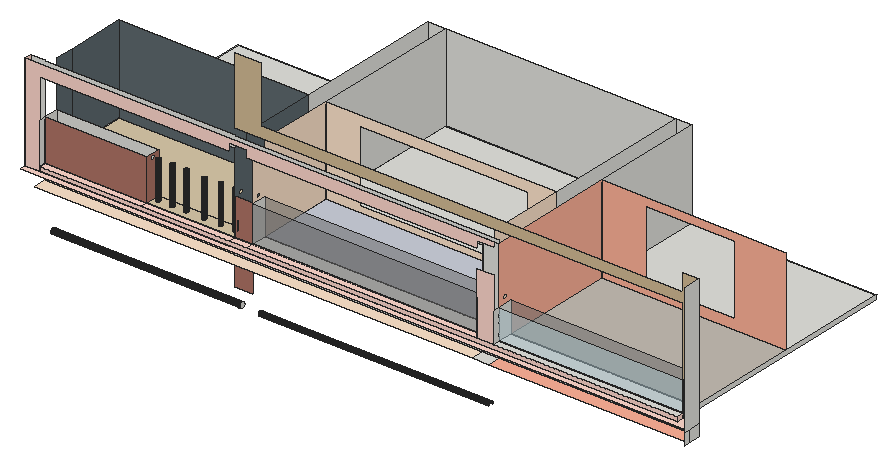
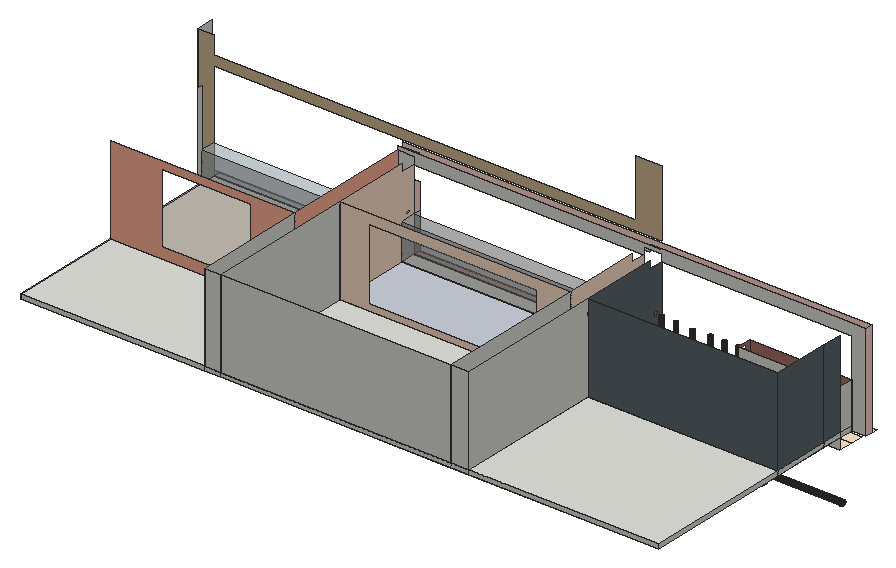
# SketchUp Ruby script. Lengths in inches.
U = 1.inch
M = Sketchup.active_model
def pt(a) = Geom::Point3d.new(a.map { |v| v * U })
def face(e, loops, mat)
  f = e.add_face(loops[0].map { |a| pt(a) })
  loops[1..].each { |l| e.add_face(l.map { |a| pt(a) }).erase! }
  f.material = f.back_material = mat if mat
  f
end
# faces: each face lists its corners as indices into pts; further lists are holes
def faces(e, pts, list, mat = nil) = list.each { |f| face(e, (f[0].is_a?(Array) ? f : [f]).map { |l| l.map { |i| pts[i] } }, mat) }
# xy, xz, yz: faces in a plane at the given z, y or x. An outline is a flat list of corners, or four numbers for a rectangle; further outlines are holes
def ring(l) = l.size == 4 ? [[l[0], l[1]], [l[2], l[1]], [l[2], l[3]], [l[0], l[3]]] : l.each_slice(2).to_a
def flat(e, list, mat, &to3) = list.each { |f| face(e, (f[0].is_a?(Array) ? f : [f]).map { |l| ring(l).map { |u, v| to3.(u, v) } }, mat) }
def xy(e, z, list, mat = nil) = flat(e, list, mat) { |x, y| [x, y, z] }
def xz(e, y, list, mat = nil) = flat(e, list, mat) { |x, z| [x, y, z] }
def yz(e, x, list, mat = nil) = flat(e, list, mat) { |y, z| [x, y, z] }
def lines(e, pts, list) = list.each { |a, b| e.add_line(pt(pts[a]), pt(pts[b])) }
# prism: a flat outline (further loops are holes) pulled along v
def prism(e, loops, v, mat = nil)
  f = face(e, loops, mat); d = Geom::Vector3d.new(v.map { |x| x * U })
  f.pushpull(f.normal.samedirection?(d) ? d.length : -d.length)
end
def box(e, o, s, mat = nil) = prism(e, [[o, [o[0] + s[0], o[1], o[2]], [o[0] + s[0], o[1] + s[1], o[2]], [o[0], o[1] + s[1], o[2]]]], [0, 0, s[2]], mat)
def at(x, y, z, deg = 0) = Geom::Transformation.translation(pt([x, y, z])) * Geom::Transformation.rotation(ORIGIN, Z_AXIS, deg.degrees)
def axes(o, x, y, z) = Geom::Transformation.new([*x, 0, *y, 0, *z, 0, *pt(o).to_a, 1])
def part(name) = M.definitions.add(name)
# library, detail: a bought-in or finely detailed component or shape, given as its bounding box
def library(name, o, s) = part(name).tap { |d| box(d.entities, o, s) }
def detail(e, o, s) = box(e.add_group.entities, o, s)
def put(e, d, t, mat = nil) = e.add_instance(d, t).tap { |i| i.material = mat if mat }
def group(e, t, mat = nil) = e.add_group.tap { |g| g.transformation = t; g.material = mat if mat }.entities
root = M.entities
M.materials.add("[Color B01]").color = [255, 216, 204]
M.materials.add("[Color B02]").color = [255, 178, 153]
M.materials.add("[Color C01]").color = [255, 229, 204]
M.materials.add("[Field Rectangle Tile]").color = [196, 189, 179]
M.materials.add("[Field Square Tile]").color = [217, 201, 169]
M.materials.add("[Formica Beige]").color = [211, 187, 149]
M.materials.add("[Formica Graystone]").color = [149, 146, 135]
M.materials.add("[Formica Laminate Dark]").color = [50, 53, 60]
M.materials.add("[Formica Speckled Grey]").color = [94, 105, 111]
M.materials.add("[Marble Carrara Floor Tile]").color = [204, 208, 219]
M.materials.add("[Stone Flagstone Ashlar]").color = [175, 116, 102]
M.materials.add("[Stone Flagstone Ashlar]1").color = [175, 116, 102]
M.materials.add("[Terrazzo Tile Light]").color = [219, 217, 210]
M.materials.add("[Translucent Glass Gray]").color = [128, 128, 128]
M.materials["[Translucent Glass Gray]"].alpha = 0.5
M.materials.add("[Translucent Glass Safety]").color = [204, 235, 244]
M.materials["[Translucent Glass Safety]"].alpha = 0.5
M.materials.add("[Wood Veneer 01]").color = [76, 44, 23]
xy(root,2054.4,[[2080.39,1246.93,2186.14,1258.93],[2207.95,1246.93,2312.17,1258.93]])
xy(root,2071.89,[[2062.91,1246.93,2329.66,1258.93]],"[Formica Laminate Dark]")
xy(root,2074.78,[[727.84,1144.55,801.89,1156.55],[817.41,1144.55,895.77,1156.55]])
xy(root,2077.28,[[1321.97,1144.55,1448.68,1156.55],[1465.17,1144.55,1591.81,1156.55],[1608.29,1144.55,1721.62,1156.55],[1738.1,1144.55,1854.25,1156.55]],"[Wood Veneer 01]")
xy(root,2083.5625,[[1905.54,863.74,1950.59,899.87]])
xy(root,2083.5625,[[1950.59,863.74,2507.95,899.87]],"[Color B02]")
xy(root,2083.5625,[[686.75,863.74,1905.54,899.87],[686.75,899.87,1950.59,941.93]],"[Color C01]")
xy(root,2089.12,[[713.49,1144.55,910.11,1156.55]])
xy(root,2092.65,[[1306.61,1144.55,1869.61,1156.55]])
xy(root,2114.125,[[646.49,880.68,686.75,899.87],[686.75,880.68,1214.63,899.87],[1214.63,880.68,1263.92,899.87],[1263.92,880.68,1905.54,899.87],[1905.54,880.68,1950.59,899.87],
  [1950.59,880.68,2463.34,899.87],[686.75,899.87,1214.63,941.93],[1214.63,899.87,1263.92,941.93],[1263.92,899.87,1905.54,941.93],[1905.54,899.87,1950.59,941.93],
  [1214.63,941.93,1263.92,1358.15],[1905.54,941.93,1950.59,1358.15],[686.75,1156.55,1214.63,1571.68],[1263.92,1156.55,1905.54,1358.15],[1950.59,1258.93,2463.34,1358.15],
  [1214.63,1358.15,1263.92,1571.68],[1263.92,1358.15,1905.54,1571.68],[1905.54,1358.15,1950.59,1571.68],[1950.59,1358.15,2463.34,1571.68]])
xy(root,2114.125,[[646.49,863.74,2507.95,863.74,2507.95,899.87,2463.34,899.87,2463.34,880.68,646.49,880.68]],"[Color B01]")
xy(root,2114.125,[[1950.59,899.87,2463.34,1258.93]],"[Color B02]")
xy(root,2114.125,[[1263.92,941.93,1905.54,1156.55]],"[Color C01]")
xy(root,2114.125,[[686.75,941.93,1214.63,1156.55]],"[Terrazzo Tile Light]")
xy(root,2126.125,[[1905.54,880.68,1950.59,899.87],[1950.59,880.68,2463.34,899.87],[686.75,899.87,969.66,941.93],[1214.63,899.87,1263.92,1571.68],[1263.92,899.87,1905.54,941.93],
  [1905.54,899.87,1950.59,1571.68],[1950.59,899.87,2463.34,941.93],[982.87,919.11,981.55,919.29,980.31,919.8,979.25,920.61,978.43,921.68,977.92,922.91,977.75,924.24,977.92,925.57,978.43,926.8,979.25,927.86,980.31,928.68,981.55,929.1875,982.87,929.36,984.2,929.1875,985.43,928.68,986.5,927.86,987.31,926.8,987.82,925.57,988,924.24,987.82,922.91,987.31,921.68,986.5,920.61,985.43,919.8,984.2,919.29],[1021.75,919.11,1020.42,919.29,1019.18,919.8,1018.12,920.61,1017.31,921.68,1016.8,922.91,1016.62,924.24,1016.8,925.57,1017.31,926.8,1018.12,927.86,1019.18,928.68,1020.42,929.1875,1021.75,929.36,1023.07,929.1875,1024.31,928.68,1025.37,927.86,1026.18,926.8,1026.7,925.57,1026.87,924.24,1026.7,922.91,1026.18,921.68,1025.37,920.61,1024.31,919.8,1023.07,919.29],[1060.43,919.11,1059.11,919.29,1057.87,919.8,1056.81,920.61,1056,921.68,1055.48,922.91,1055.31,924.24,1055.48,925.57,1056,926.8,1056.81,927.86,1057.87,928.68,1059.11,929.1875,1060.43,929.36,1061.76,929.1875,1063,928.68,1064.06,927.86,1064.87,926.8,1065.38,925.57,1065.56,924.24,1065.38,922.91,1064.87,921.68,1064.06,920.61,1063,919.8,1061.76,919.29],
  [1110.56,919.11,1109.23,919.29,1108,919.8,1106.94,920.61,1106.12,921.68,1105.61,922.91,1105.43,924.24,1105.61,925.57,1106.12,926.8,1106.94,927.86,1108,928.68,1109.23,929.1875,1110.56,929.36,1111.89,929.1875,1113.12,928.68,1114.18,927.86,1115,926.8,1115.51,925.57,1115.68,924.24,1115.51,922.91,1115,921.68,1114.18,920.61,1113.12,919.8,1111.89,919.29],[1156.68,919.11,1155.36,919.29,1154.12,919.8,1153.06,920.61,1152.25,921.68,1151.73,922.91,1151.56,924.24,1151.73,925.57,1152.25,926.8,1153.06,927.86,1154.12,928.68,1155.36,929.1875,1156.68,929.36,1158.01,929.1875,1159.25,928.68,1160.31,927.86,1161.12,926.8,1161.63,925.57,1161.81,924.24,1161.63,922.91,1161.12,921.68,1160.31,920.61,1159.25,919.8,1158.01,919.29],[1197.43,919.11,1196.11,919.29,1194.87,919.8,1193.81,920.61,1193,921.68,1192.48,922.91,1192.31,924.24,1192.48,925.57,1193,926.8,1193.81,927.86,1194.87,928.68,1196.11,929.1875,1197.43,929.36,1198.76,929.1875,1200,928.68,1201.06,927.86,1201.87,926.8,1202.38,925.57,1202.56,924.24,1202.38,922.91,1201.87,921.68,1201.06,920.61,1200,919.8,1198.76,919.29],[686.75,1156.55,1214.63,1571.68],[1263.92,1156.55,1905.54,1571.68],
  [1950.59,1258.05,2463.34,1571.68],[2463.34,1258.05,2464.28,1571.68]])
xy(root,2126.125,[[686.75,880.68,969.66,899.87],[969.66,880.68,1214.63,899.87],[1214.63,880.68,1263.92,899.87],[1263.92,880.68,1905.54,899.87]],"[Color B01]")
xy(root,2126.125,[[1950.59,941.93,2463.34,1258.05]],"[Field Rectangle Tile]")
xy(root,2126.125,[[[969.66,899.87,1214.63,941.93],[982.87,919.11,981.55,919.29,980.31,919.8,979.25,920.61,978.43,921.68,977.92,922.91,977.75,924.24,977.92,925.57,978.43,926.8,979.25,927.86,980.31,928.68,981.55,929.1875,982.87,929.36,984.2,929.1875,985.43,928.68,986.5,927.86,987.31,926.8,987.82,925.57,988,924.24,987.82,922.91,987.31,921.68,986.5,920.61,985.43,919.8,984.2,919.29],[1197.43,919.11,1196.11,919.29,1194.87,919.8,1193.81,920.61,1193,921.68,1192.48,922.91,1192.31,924.24,1192.48,925.57,1193,926.8,1193.81,927.86,1194.87,928.68,1196.11,929.1875,1197.43,929.36,1198.76,929.1875,1200,928.68,1201.06,927.86,1201.87,926.8,1202.38,925.57,1202.56,924.24,1202.38,922.91,1201.87,921.68,1201.06,920.61,1200,919.8,1198.76,919.29],[1021.75,919.11,1020.42,919.29,1019.18,919.8,1018.12,920.61,1017.31,921.68,1016.8,922.91,1016.62,924.24,1016.8,925.57,1017.31,926.8,1018.12,927.86,1019.18,928.68,1020.42,929.1875,1021.75,929.36,1023.07,929.1875,1024.31,928.68,1025.37,927.86,1026.18,926.8,1026.7,925.57,1026.87,924.24,1026.7,922.91,1026.18,921.68,1025.37,920.61,1024.31,919.8,1023.07,919.29],[1156.68,919.11,1155.36,919.29,1154.12,919.8,1153.06,920.61,1152.25,921.68,1151.73,922.91,1151.56,924.24,1151.73,925.57,1152.25,926.8,1153.06,927.86,1154.12,928.68,1155.36,929.1875,1156.68,929.36,1158.01,929.1875,1159.25,928.68,1160.31,927.86,1161.12,926.8,1161.63,925.57,1161.81,924.24,1161.63,922.91,1161.12,921.68,1160.31,920.61,1159.25,919.8,1158.01,919.29],[1060.43,919.11,1059.11,919.29,1057.87,919.8,1056.81,920.61,1056,921.68,1055.48,922.91,1055.31,924.24,1055.48,925.57,1056,926.8,1056.81,927.86,1057.87,928.68,1059.11,929.1875,1060.43,929.36,1061.76,929.1875,1063,928.68,1064.06,927.86,1064.87,926.8,1065.38,925.57,1065.56,924.24,1065.38,922.91,1064.87,921.68,1064.06,920.61,1063,919.8,1061.76,919.29],[1110.56,919.11,1109.23,919.29,1108,919.8,1106.94,920.61,1106.12,921.68,1105.61,922.91,1105.43,924.24,1105.61,925.57,1106.12,926.8,1106.94,927.86,1108,928.68,1109.23,929.1875,1110.56,929.36,1111.89,929.1875,1113.12,928.68,1114.18,927.86,1115,926.8,1115.51,925.57,1115.68,924.24,1115.51,922.91,1115,921.68,1114.18,920.61,1113.12,919.8,1111.89,919.29]],[686.75,941.93,1214.63,1156.55]],"[Field Square Tile]")
xy(root,2126.125,[[1263.92,941.93,1905.54,1156.55]],"[Marble Carrara Floor Tile]")
xz(root,880.68,[[646.49,2114.125,686.75,2114.125,686.75,2350.0625,1214.63,2350.0625,1214.63,2369.6875,1263.92,2369.6875,1263.92,2350.0625,1905.54,2350.0625,1905.54,2369.6875,1950.59,2369.6875,1950.59,2383.06,646.49,2383.06],[686.75,2114.125,2463.34,2126.125],[1905.54,2126.125,1950.59,2298.64]],"[Color B01]")
xz(root,899.87,[[1214.63,2083.5625,1263.92,2114.125],[1263.92,2083.5625,1905.54,2114.125],[1905.54,2083.5625,1950.59,2114.125],[1950.59,2083.5625,2463.34,2114.125],[2463.34,2083.5625,2507.95,2114.125],
  [646.49,2114.125,646.49,2383.06,686.75,2383.06,686.75,2381.6875,1215.84,2381.6875,1215.84,2379.45,1950.59,2379.45,1950.59,2369.6875,1905.54,2369.6875,1905.54,2350.0625,1263.92,2350.0625,1263.92,2369.6875,1214.63,2369.6875,1214.63,2350.0625,686.75,2350.0625,686.75,2114.125],[686.75,2114.125,2463.34,2126.125],[1905.54,2126.125,1950.59,2369.6875]])
xz(root,899.87,[[2463.34,2114.125,2507.95,2114.125,2507.95,2476.875,2463.34,2476.875,2463.34,2428.82,1286.83,2428.82,1286.83,2588.07,1215.84,2588.07,1215.84,2400.95,2463.34,2400.95]],"[Formica Beige]")
xz(root,899.87,[[686.75,2126.125,969.66,2241]],"[Stone Flagstone Ashlar]")
xz(root,899.87,[[1214.63,2003.5,1263.92,2083.5625],[1214.63,2126.125,1263.92,2230.66]],"[Stone Flagstone Ashlar]1")
xz(root,899.87,[[1263.92,2126.125,1905.54,2226.5]],"[Translucent Glass Gray]")
xz(root,899.87,[[1950.59,2126.125,2463.34,2209.0625]],"[Translucent Glass Safety]")
xz(root,941.93,[[686.75,2083.5625,1950.59,2114.125],[686.75,2126.125,969.66,2241]])
xz(root,941.93,[[1263.92,2126.125,1905.54,2226.5],[1950.59,2126.125,2463.34,2209.0625]],"[Translucent Glass Gray]")
xz(root,1156.55,[[[1263.92,2126.125,1905.54,2369.6875],[1358.7,2142.09,1824.89,2342.28]]],"[Color C01]")
xz(root,1156.55,[[686.75,2126.125,1214.63,2369.6875]],"[Formica Speckled Grey]")
xz(root,1258.05,[[[1950.59,2126.125,2464.28,2369.6875],[2073.08,2155.2,2321.89,2349.01]]],"[Color B02]")
xz(root,1571.68,[[686.75,2114.125,1214.63,2126.125],[1214.63,2114.125,1263.92,2126.125],[1263.92,2114.125,1905.54,2126.125],[1905.54,2114.125,1950.59,2126.125],[1950.59,2114.125,2463.34,2126.125],
  [1214.63,2126.125,1263.92,2369.6875],[1263.92,2126.125,1905.54,2369.6875],[1905.54,2126.125,1950.59,2369.6875]])
yz(root,646.49,[[880.68,2114.125,899.87,2383.06]],"[Color B01]")
yz(root,686.75,[[880.68,2114.125,899.87,2126.125],[899.87,2114.125,941.93,2126.125],[941.93,2114.125,994.87,2126.125],[994.87,2114.125,1156.55,2126.125],[1156.55,2114.125,1571.68,2126.125],
  [880.68,2126.125,899.87,2241],[899.87,2126.125,941.93,2241]])
yz(root,686.75,[[941.93,2126.125,994.87,2369.6875],[994.87,2126.125,1156.55,2369.6875]],"[Formica Speckled Grey]")
yz(root,969.66,[[[899.87,2126.125,941.93,2241],[921.12,2224.46,919.47,2224.68,917.93,2225.3125,916.61,2226.33,915.6,2227.65,914.96,2229.19,914.74,2230.84,914.96,2232.49,915.6,2234.02,916.61,2235.34,917.93,2236.36,919.47,2236.99,921.12,2237.21,922.77,2236.99,924.3,2236.36,925.625,2235.34,926.64,2234.02,927.27,2232.49,927.49,2230.84,927.27,2229.19,926.64,2227.65,925.625,2226.33,924.3,2225.3125,922.77,2224.68]]],"[Stone Flagstone Ashlar]")
yz(root,1214.63,[[927.21,1938.33,928.92,1938.56,930.51,1939.22,931.88,1940.26,932.93,1941.63,933.59,1943.22,933.8125,1944.93,933.59,1946.64,932.93,1948.23,931.88,1949.6,930.51,1950.65,928.92,1951.31,927.21,1951.53,925.5,1951.31,923.91,1950.65,922.55,1949.6,921.5,1948.23,920.84,1946.64,920.61,1944.93,920.84,1943.22,921.5,1941.63,922.55,1940.26,923.91,1939.22,925.5,1938.56],[1156.55,2126.125,1571.68,2369.6875]])
yz(root,1214.63,[[[899.87,2126.125,899.87,2350.0625,941.93,2350.0625,941.93,2369.6875,1156.55,2369.6875,1156.55,2126.125],[921.12,2224.46,922.77,2224.68,924.3,2225.3125,925.625,2226.33,926.64,2227.65,927.27,2229.19,927.49,2230.84,927.27,2232.49,926.64,2234.02,925.625,2235.34,924.3,2236.36,922.77,2236.99,921.12,2237.21,919.47,2236.99,917.93,2236.36,916.61,2235.34,915.6,2234.02,914.96,2232.49,914.74,2230.84,914.96,2229.19,915.6,2227.65,916.61,2226.33,917.93,2225.3125,919.47,2224.68]]],"[Formica Speckled Grey]")
yz(root,1263.92,[[899.87,2126.125,941.93,2226.5],[1156.55,2126.125,1571.68,2369.6875]])
yz(root,1263.92,[[[941.93,2126.125,1156.55,2126.125,1156.55,2369.6875,941.93,2369.6875,941.93,2350.0625,899.87,2350.0625,899.87,2226.5,941.93,2226.5],[920.9,2234.39,919.46,2234.58,918.12,2235.14,916.97,2236.02,916.08,2237.18,915.53,2238.52,915.34,2239.96,915.53,2241.4,916.08,2242.74,916.97,2243.89,918.12,2244.77,919.46,2245.33,920.9,2245.52,922.34,2245.33,923.68,2244.77,924.83,2243.89,925.72,2242.74,926.27,2241.4,926.46,2239.96,926.27,2238.52,925.72,2237.18,924.83,2236.02,923.68,2235.14,922.34,2234.58]]],"[Color C01]")
yz(root,1905.54,[[880.68,2126.125,899.87,2226.5],[899.87,2126.125,941.93,2226.5],[1156.55,2126.125,1571.68,2369.6875]])
yz(root,1905.54,[[[941.93,2126.125,941.93,2226.5,899.87,2226.5,899.87,2350.0625,941.93,2350.0625,941.93,2369.6875,1156.55,2369.6875,1156.55,2126.125],[920.9,2234.39,922.34,2234.58,923.68,2235.14,924.83,2236.02,925.72,2237.18,926.27,2238.52,926.46,2239.96,926.27,2241.4,925.72,2242.74,924.83,2243.89,923.68,2244.77,922.34,2245.33,920.9,2245.52,919.46,2245.33,918.12,2244.77,916.97,2243.89,916.08,2242.74,915.53,2241.4,915.34,2239.96,915.53,2238.52,916.08,2237.18,916.97,2236.02,918.12,2235.14,919.46,2234.58]]],"[Color C01]")
yz(root,1950.59,[[899.87,2083.5625,941.93,2114.125],[880.68,2126.125,899.87,2209.0625],[899.87,2126.125,941.93,2209.0625],[1258.05,2126.125,1571.68,2369.6875]])
yz(root,1950.59,[[[941.93,2126.125,1258.05,2126.125,1258.05,2369.6875,899.87,2369.6875,899.87,2209.0625,941.93,2209.0625],[920.9,2220.96,919.11,2221.2,917.43,2221.89,916,2222.99,914.89,2224.43,914.2,2226.1,913.96,2227.9,914.2,2229.69,914.89,2231.37,916,2232.8,917.43,2233.91,919.11,2234.6,920.9,2234.84,922.7,2234.6,924.37,2233.91,925.81,2232.8,926.91,2231.37,927.6,2229.69,927.84,2227.9,927.6,2226.1,926.91,2224.43,925.81,2222.99,924.37,2221.89,922.7,2221.2]]],"[Color B02]")
yz(root,2463.34,[[899.87,2114.125,941.93,2126.125],[941.93,2114.125,954.56,2126.125],[954.56,2114.125,1571.68,2126.125],[899.87,2126.125,941.93,2209.0625],[941.93,2126.125,954.56,2369.6875]])
yz(root,2463.34,[[880.68,2114.125,899.87,2126.125]],"[Color B01]")
yz(root,2507.95,[[849.3125,2083.5625,863.74,2114.125],[863.74,2083.5625,899.87,2114.125],[849.3125,2114.125,899.87,2476.875]])
p = [[1214.63,927.21,1938.33],[1214.63,925.5,1938.56],[686.75,925.5,1938.56],[686.75,927.21,1938.33],[1214.63,928.92,1938.56],[686.75,928.92,1938.56],
  [1214.63,923.91,1939.22],[686.75,923.91,1939.22],[1214.63,930.51,1939.22],[686.75,930.51,1939.22],[1905.54,920.8125,1939.12],[1905.54,920.59,1940.84],
  [1263.92,920.59,1940.84],[1263.92,920.8125,1939.12],[1905.54,933.84,1940.84],[1905.54,933.61,1939.12],[1263.92,933.61,1939.12],[1263.92,933.84,1940.84],
  [1214.63,922.55,1940.26],[686.75,922.55,1940.26],[1214.63,931.88,1940.26],[686.75,931.88,1940.26],[1214.63,921.5,1941.63],[686.75,921.5,1941.63],
  [1214.63,932.93,1941.63],[686.75,932.93,1941.63],[1905.54,920.8125,1942.55],[1263.92,920.8125,1942.55],[1905.54,933.61,1942.55],[1263.92,933.61,1942.55],
  [1214.63,920.84,1943.22],[686.75,920.84,1943.22],[1214.63,933.59,1943.22],[686.75,933.59,1943.22],[1905.54,921.48,1944.15],[1263.92,921.48,1944.15],
  [1905.54,932.95,1944.15],[1263.92,932.95,1944.15],[1214.63,920.61,1944.93],[686.75,920.61,1944.93],[1214.63,933.8125,1944.93],[686.75,933.8125,1944.93],
  [1905.54,922.53,1945.52],[1263.92,922.53,1945.52],[1905.54,931.9,1945.52],[1263.92,931.9,1945.52],[1214.63,920.84,1946.64],[686.75,920.84,1946.64],
  [1214.63,933.59,1946.64],[686.75,933.59,1946.64],[1905.54,923.9,1946.57],[1263.92,923.9,1946.57],[1905.54,930.53,1946.57],[1263.92,930.53,1946.57],
  [1214.63,921.5,1948.23],[686.75,921.5,1948.23],[1905.54,925.5,1947.24],[1263.92,925.5,1947.24],[1905.54,928.93,1947.24],[1263.92,928.93,1947.24],
  [1214.63,932.93,1948.23],[686.75,932.93,1948.23],[1905.54,927.21,1947.46],[1263.92,927.21,1947.46],[1214.63,922.55,1949.6],[686.75,922.55,1949.6],
  [1214.63,931.88,1949.6],[686.75,931.88,1949.6],[1214.63,923.91,1950.65],[686.75,923.91,1950.65],[1214.63,930.51,1950.65],[686.75,930.51,1950.65],
  [1214.63,925.5,1951.31],[686.75,925.5,1951.31],[1214.63,928.92,1951.31],[686.75,928.92,1951.31],[1214.63,927.21,1951.53],[686.75,927.21,1951.53],
  [981.55,919.29,2126.125],[982.87,919.11,2126.125],[982.87,919.11,2230.84],[981.55,919.29,2230.84],[984.2,919.29,2126.125],[984.2,919.29,2230.84],
  [1020.42,919.29,2126.125],[1021.75,919.11,2126.125],[1021.75,919.11,2230.84],[1020.42,919.29,2230.84],[1023.07,919.29,2126.125],[1023.07,919.29,2230.84],
  [1059.11,919.29,2126.125],[1060.43,919.11,2126.125],[1060.43,919.11,2230.84],[1059.11,919.29,2230.84],[1061.76,919.29,2126.125],[1061.76,919.29,2230.84],
  [1109.23,919.29,2126.125],[1110.56,919.11,2126.125],[1110.56,919.11,2228],[1109.23,919.29,2228],[1111.89,919.29,2126.125],[1111.89,919.29,2228],
  [1155.36,919.29,2126.125],[1156.68,919.11,2126.125],[1156.68,919.11,2230.84],[1155.36,919.29,2230.84],[1158.01,919.29,2126.125],[1158.01,919.29,2230.84],
  [1196.11,919.29,2126.125],[1197.43,919.11,2126.125],[1197.43,919.11,2232],[1196.11,919.29,2232],[1198.76,919.29,2126.125],[1198.76,919.29,2232],
  [980.31,919.8,2126.125],[980.31,919.8,2230.84],[985.43,919.8,2126.125],[985.43,919.8,2230.84],[1019.18,919.8,2126.125],[1019.18,919.8,2230.84],
  [1024.31,919.8,2126.125],[1024.31,919.8,2230.84],[1057.87,919.8,2126.125],[1057.87,919.8,2230.84],[1063,919.8,2126.125],[1063,919.8,2230.84],
  [1108,919.8,2126.125],[1108,919.8,2228],[1113.12,919.8,2126.125],[1113.12,919.8,2228],[1154.12,919.8,2126.125],[1154.12,919.8,2230.84],
  [1159.25,919.8,2126.125],[1159.25,919.8,2230.84],[1194.87,919.8,2126.125],[1194.87,919.8,2232],[1200,919.8,2126.125],[1200,919.8,2232],
  [979.25,920.61,2126.125],[979.25,920.61,2230.84],[986.5,920.61,2126.125],[986.5,920.61,2230.84],[1018.12,920.61,2126.125],[1018.12,920.61,2230.84],
  [1025.37,920.61,2126.125],[1025.37,920.61,2230.84],[1056.81,920.61,2126.125],[1056.81,920.61,2230.84],[1064.06,920.61,2126.125],[1064.06,920.61,2230.84],
  [1106.94,920.61,2126.125],[1106.94,920.61,2228],[1114.18,920.61,2126.125],[1114.18,920.61,2228],[1153.06,920.61,2126.125],[1153.06,920.61,2230.84],
  [1160.31,920.61,2126.125],[1160.31,920.61,2230.84],[1193.81,920.61,2126.125],[1193.81,920.61,2232],[1201.06,920.61,2126.125],[1201.06,920.61,2232],
  [978.43,921.68,2126.125],[978.43,921.68,2230.84],[987.31,921.68,2126.125],[987.31,921.68,2230.84],[1017.31,921.68,2126.125],[1017.31,921.68,2230.84],
  [1026.18,921.68,2126.125],[1026.18,921.68,2230.84],[1056,921.68,2126.125],[1056,921.68,2230.84],[1064.87,921.68,2126.125],[1064.87,921.68,2230.84],
  [1106.12,921.68,2126.125],[1106.12,921.68,2228],[1115,921.68,2126.125],[1115,921.68,2228],[1152.25,921.68,2126.125],[1152.25,921.68,2230.84],
  [1161.12,921.68,2126.125],[1161.12,921.68,2230.84],[1193,921.68,2126.125],[1193,921.68,2232],[1201.87,921.68,2126.125],[1201.87,921.68,2232],
  [977.92,922.91,2126.125],[977.92,922.91,2230.84],[987.82,922.91,2126.125],[987.82,922.91,2230.84],[1016.8,922.91,2126.125],[1016.8,922.91,2230.84],
  [1026.7,922.91,2126.125],[1026.7,922.91,2230.84],[1055.48,922.91,2126.125],[1055.48,922.91,2230.84],[1065.38,922.91,2126.125],[1065.38,922.91,2230.84],
  [1105.61,922.91,2126.125],[1105.61,922.91,2228],[1115.51,922.91,2126.125],[1115.51,922.91,2228],[1151.73,922.91,2126.125],[1151.73,922.91,2230.84],
  [1161.63,922.91,2126.125],[1161.63,922.91,2230.84],[1192.48,922.91,2126.125],[1192.48,922.91,2232],[1202.38,922.91,2126.125],[1202.38,922.91,2232],
  [977.75,924.24,2126.125],[977.75,924.24,2230.84],[988,924.24,2126.125],[988,924.24,2230.84],[1016.62,924.24,2126.125],[1016.62,924.24,2230.84],
  [1026.87,924.24,2126.125],[1026.87,924.24,2230.84],[1055.31,924.24,2126.125],[1055.31,924.24,2230.84],[1065.56,924.24,2126.125],[1065.56,924.24,2230.84],
  [1105.43,924.24,2126.125],[1105.43,924.24,2228],[1115.68,924.24,2126.125],[1115.68,924.24,2228],[1151.56,924.24,2126.125],[1151.56,924.24,2230.84],
  [1161.81,924.24,2126.125],[1161.81,924.24,2230.84],[1192.31,924.24,2126.125],[1192.31,924.24,2232],[1202.56,924.24,2126.125],[1202.56,924.24,2232],
  [977.92,925.57,2126.125],[977.92,925.57,2230.84],[987.82,925.57,2126.125],[987.82,925.57,2230.84],[1016.8,925.57,2126.125],[1016.8,925.57,2230.84],
  [1026.7,925.57,2126.125],[1026.7,925.57,2230.84],[1055.48,925.57,2126.125],[1055.48,925.57,2230.84],[1065.38,925.57,2126.125],[1065.38,925.57,2230.84],
  [1105.61,925.57,2126.125],[1105.61,925.57,2228],[1115.51,925.57,2126.125],[1115.51,925.57,2228],[1151.73,925.57,2126.125],[1151.73,925.57,2230.84],
  [1161.63,925.57,2126.125],[1161.63,925.57,2230.84],[1192.48,925.57,2126.125],[1192.48,925.57,2232],[1202.38,925.57,2126.125],[1202.38,925.57,2232],
  [978.43,926.8,2126.125],[978.43,926.8,2230.84],[987.31,926.8,2126.125],[987.31,926.8,2230.84],[1017.31,926.8,2126.125],[1017.31,926.8,2230.84],
  [1026.18,926.8,2126.125],[1026.18,926.8,2230.84],[1056,926.8,2126.125],[1056,926.8,2230.84],[1064.87,926.8,2126.125],[1064.87,926.8,2230.84],
  [1106.12,926.8,2126.125],[1106.12,926.8,2228],[1115,926.8,2126.125],[1115,926.8,2228],[1152.25,926.8,2126.125],[1152.25,926.8,2230.84],
  [1161.12,926.8,2126.125],[1161.12,926.8,2230.84],[1193,926.8,2126.125],[1193,926.8,2232],[1201.87,926.8,2126.125],[1201.87,926.8,2232],
  [979.25,927.86,2126.125],[978.96,927.49,2230.84],[979.25,927.86,2230.84],[986.5,927.86,2126.125],[986.5,927.86,2230.84],[986.78,927.49,2230.84],
  [1018.12,927.86,2126.125],[1017.84,927.49,2230.84],[1018.12,927.86,2230.84],[1025.37,927.86,2126.125],[1025.37,927.86,2230.84],[1025.66,927.49,2230.84],
  [1056.81,927.86,2126.125],[1056.53,927.49,2230.84],[1056.81,927.86,2230.84],[1064.06,927.86,2126.125],[1064.06,927.86,2230.84],[1064.34,927.49,2230.84],
  [1106.94,927.86,2126.125],[1106.94,927.86,2228],[1114.18,927.86,2126.125],[1114.18,927.86,2228],[1153.06,927.86,2126.125],[1152.78,927.49,2230.84],
  [1153.06,927.86,2230.84],[1160.31,927.86,2126.125],[1160.31,927.86,2230.84],[1160.59,927.49,2230.84],[1193.81,927.86,2126.125],[1193.81,927.86,2232],
  [1201.06,927.86,2126.125],[1201.06,927.86,2232],[980.31,928.68,2126.125],[980.31,928.68,2230.84],[985.43,928.68,2126.125],[985.43,928.68,2230.84],
  [1019.18,928.68,2126.125],[1019.18,928.68,2230.84],[1024.31,928.68,2126.125],[1024.31,928.68,2230.84],[1057.87,928.68,2126.125],[1057.87,928.68,2230.84],
  [1063,928.68,2126.125],[1063,928.68,2230.84],[1108,928.68,2126.125],[1108,928.68,2228],[1113.12,928.68,2126.125],[1113.12,928.68,2228],
  [1154.12,928.68,2126.125],[1154.12,928.68,2230.84],[1159.25,928.68,2126.125],[1159.25,928.68,2230.84],[1194.87,928.68,2126.125],[1194.87,928.68,2232],
  [1200,928.68,2126.125],[1200,928.68,2232],[981.55,929.1875,2126.125],[981.55,929.1875,2230.84],[984.2,929.1875,2126.125],[984.2,929.1875,2230.84],
  [1020.42,929.1875,2126.125],[1020.42,929.1875,2230.84],[1023.07,929.1875,2126.125],[1023.07,929.1875,2230.84],[1059.11,929.1875,2126.125],[1059.11,929.1875,2230.84],
  [1061.76,929.1875,2126.125],[1061.76,929.1875,2230.84],[1109.23,929.1875,2126.125],[1109.23,929.1875,2228],[1111.89,929.1875,2126.125],[1111.89,929.1875,2228],
  [1155.36,929.1875,2126.125],[1155.36,929.1875,2230.84],[1158.01,929.1875,2126.125],[1158.01,929.1875,2230.84],[1196.11,929.1875,2126.125],[1196.11,929.1875,2232],
  [1198.76,929.1875,2126.125],[1198.76,929.1875,2232],[982.87,929.36,2126.125],[982.87,929.36,2230.84],[1021.75,929.36,2126.125],[1021.75,929.36,2230.84],
  [1060.43,929.36,2126.125],[1060.43,929.36,2230.84],[1110.56,929.36,2126.125],[1110.56,929.36,2228],[1156.68,929.36,2126.125],[1156.68,929.36,2230.84],
  [1197.43,929.36,2126.125],[1197.43,929.36,2232]]
faces(root,p,[[0,1,2,3],[4,0,3,5],[1,6,7,2],[8,4,5,9],[10,11,12,13],[14,15,16,17],[6,18,19,7],[20,8,9,21],
  [18,22,23,19],[24,20,21,25],[11,26,27,12],[28,14,17,29],[22,30,31,23],[32,24,25,33],[26,34,35,27],[36,28,29,37],
  [30,38,39,31],[40,32,33,41],[34,42,43,35],[44,36,37,45],[38,46,47,39],[48,40,41,49],[42,50,51,43],[52,44,45,53],
  [46,54,55,47],[50,56,57,51],[58,52,53,59],[60,48,49,61],[56,62,63,57],[62,58,59,63],[54,64,65,55],[66,60,61,67],
  [64,68,69,65],[70,66,67,71],[68,72,73,69],[74,70,71,75],[72,76,77,73],[76,74,75,77]],"[Formica Laminate Dark]")
faces(root,p,[[78,79,80,81],[79,82,83,80],[84,85,86,87],[85,88,89,86],[90,91,92,93],[91,94,95,92],[96,97,98,99],[97,100,101,98],
  [102,103,104,105],[103,106,107,104],[108,109,110,111],[109,112,113,110],[114,78,81,115],[82,116,117,83],[118,84,87,119],[88,120,121,89],
  [122,90,93,123],[94,124,125,95],[126,96,99,127],[100,128,129,101],[130,102,105,131],[106,132,133,107],[134,108,111,135],[112,136,137,113],
  [138,114,115,139],[116,140,141,117],[142,118,119,143],[120,144,145,121],[146,122,123,147],[124,148,149,125],[150,126,127,151],[128,152,153,129],
  [154,130,131,155],[132,156,157,133],[158,134,135,159],[136,160,161,137],[162,138,139,163],[140,164,165,141],[166,142,143,167],[144,168,169,145],
  [170,146,147,171],[148,172,173,149],[174,150,151,175],[152,176,177,153],[178,154,155,179],[156,180,181,157],[182,158,159,183],[160,184,185,161],
  [186,162,163,187],[164,188,189,165],[190,166,167,191],[168,192,193,169],[194,170,171,195],[172,196,197,173],[198,174,175,199],[176,200,201,177],
  [202,178,179,203],[180,204,205,181],[206,182,183,207],[184,208,209,185],[210,186,187,211],[188,212,213,189],[214,190,191,215],[192,216,217,193],
  [218,194,195,219],[196,220,221,197],[222,198,199,223],[200,224,225,201],[226,202,203,227],[204,228,229,205],[230,206,207,231],[208,232,233,209],
  [234,210,211,235],[212,236,237,213],[238,214,215,239],[216,240,241,217],[242,218,219,243],[220,244,245,221],[246,222,223,247],[224,248,249,225],
  [250,226,227,251],[228,252,253,229],[254,230,231,255],[232,256,257,233],[258,234,235,259],[236,260,261,237],[262,238,239,263],[240,264,265,241],
  [266,242,243,267],[244,268,269,245],[270,246,247,271],[248,272,273,249],[274,250,251,275],[252,276,277,253],[278,254,255,279],[256,280,281,257],
  [282,258,259,283,284],[260,285,286,287,261],[288,262,263,289,290],[264,291,292,293,265],[294,266,267,295,296],[268,297,298,299,269],[300,270,271,301],[272,302,303,273],
  [304,274,275,305,306],[276,307,308,309,277],[310,278,279,311],[280,312,313,281],[314,282,284,315],[285,316,317,286],[318,288,290,319],[291,320,321,292],
  [322,294,296,323],[297,324,325,298],[326,300,301,327],[302,328,329,303],[330,304,306,331],[307,332,333,308],[334,310,311,335],[312,336,337,313],
  [338,314,315,339],[316,340,341,317],[342,318,319,343],[320,344,345,321],[346,322,323,347],[324,348,349,325],[350,326,327,351],[328,352,353,329],
  [354,330,331,355],[332,356,357,333],[358,334,335,359],[336,360,361,337],[362,338,339,363],[340,362,363,341],[364,342,343,365],[344,364,365,345],
  [366,346,347,367],[348,366,367,349],[368,350,351,369],[352,368,369,353],[370,354,355,371],[356,370,371,357],[372,358,359,373],[360,372,373,361]],"[Formica Graystone]")
